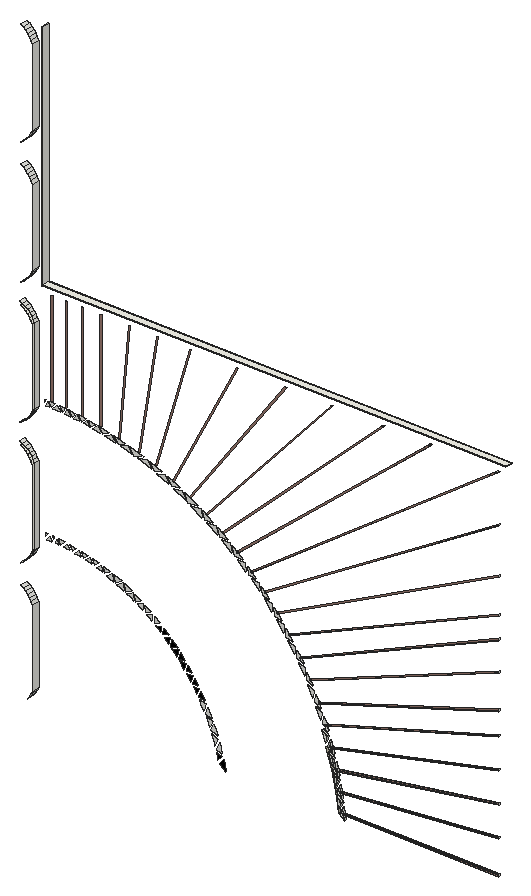
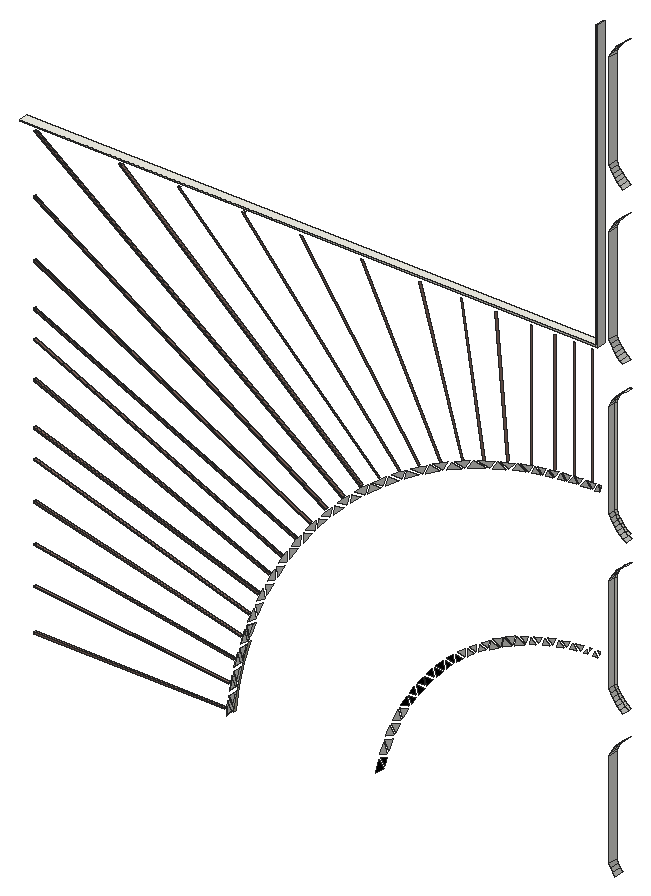
# SketchUp Ruby script. Lengths in inches.
U = 1.inch
M = Sketchup.active_model
def pt(a) = Geom::Point3d.new(a.map { |v| v * U })
def face(e, loops, mat)
  f = e.add_face(loops[0].map { |a| pt(a) })
  loops[1..].each { |l| e.add_face(l.map { |a| pt(a) }).erase! }
  f.material = f.back_material = mat if mat
  f
end
# faces: each face lists its corners as indices into pts; further lists are holes
def faces(e, pts, list, mat = nil) = list.each { |f| face(e, (f[0].is_a?(Array) ? f : [f]).map { |l| l.map { |i| pts[i] } }, mat) }
# xy, xz, yz: faces in a plane at the given z, y or x. An outline is a flat list of corners, or four numbers for a rectangle; further outlines are holes
def ring(l) = l.size == 4 ? [[l[0], l[1]], [l[2], l[1]], [l[2], l[3]], [l[0], l[3]]] : l.each_slice(2).to_a
def flat(e, list, mat, &to3) = list.each { |f| face(e, (f[0].is_a?(Array) ? f : [f]).map { |l| ring(l).map { |u, v| to3.(u, v) } }, mat) }
def xy(e, z, list, mat = nil) = flat(e, list, mat) { |x, y| [x, y, z] }
def xz(e, y, list, mat = nil) = flat(e, list, mat) { |x, z| [x, y, z] }
def yz(e, x, list, mat = nil) = flat(e, list, mat) { |y, z| [x, y, z] }
def lines(e, pts, list) = list.each { |a, b| e.add_line(pt(pts[a]), pt(pts[b])) }
# prism: a flat outline (further loops are holes) pulled along v
def prism(e, loops, v, mat = nil)
  f = face(e, loops, mat); d = Geom::Vector3d.new(v.map { |x| x * U })
  f.pushpull(f.normal.samedirection?(d) ? d.length : -d.length)
end
def box(e, o, s, mat = nil) = prism(e, [[o, [o[0] + s[0], o[1], o[2]], [o[0] + s[0], o[1] + s[1], o[2]], [o[0], o[1] + s[1], o[2]]]], [0, 0, s[2]], mat)
def at(x, y, z, deg = 0) = Geom::Transformation.translation(pt([x, y, z])) * Geom::Transformation.rotation(ORIGIN, Z_AXIS, deg.degrees)
def axes(o, x, y, z) = Geom::Transformation.new([*x, 0, *y, 0, *z, 0, *pt(o).to_a, 1])
def part(name) = M.definitions.add(name)
# library, detail: a bought-in or finely detailed component or shape, given as its bounding box
def library(name, o, s) = part(name).tap { |d| box(d.entities, o, s) }
def detail(e, o, s) = box(e.add_group.entities, o, s)
def put(e, d, t, mat = nil) = e.add_instance(d, t).tap { |i| i.material = mat if mat }
def group(e, t, mat = nil) = e.add_group.tap { |g| g.transformation = t; g.material = mat if mat }.entities
root = M.entities
M.materials.add("Tafisa-Gardenia-or-Gardenia-PM775-4K").color = [246, 245, 235]
M.materials.add("Tafisa-Terrarossa-PM780-4K").color = [148, 117, 107]
M.materials.add("Uniboard-L19-Putty-4K").color = [187, 181, 160]
M.materials.add("[Color M09]").color = [0, 0, 0]
xy(root,51.83,[[131.885,138,147.791,138.157]],"Tafisa-Terrarossa-PM780-4K")
xy(root,51.949,[[131.874,138,147.791,138.157]],"Tafisa-Terrarossa-PM780-4K")
xy(root,89.291,[[130.345,138,130.503,138.157],[135.69,138,135.862,138.157],[140.566,138,140.748,138.157],[147.588,138,147.791,138.157]])
xy(root,90,[[100.618,138,148.5,138.709]],"Uniboard-L19-Putty-4K")
xy(root,90.118,[[100.618,138,148.5,138.709]],"Tafisa-Gardenia-or-Gardenia-PM775-4K")
xz(root,138.157,[[131.8,51.347,131.745,51.932,131.653,52.513,131.327,51.879],[131.234,52.254,131.567,52.902,131.05,53.415],[119.016,52.974,118.749,53.891,118.748,53.897,118.429,53.195],[131.537,53.282,131.442,53.88,131.31,54.471,131.016,53.799],[118.288,53.48,118.6,54.168,117.933,54.514,118.219,53.719],
  [130.906,54.168,131.198,54.835,130.65,55.315],[118.539,54.477,118.344,55.018,118.178,55.401,117.877,54.82],[117.721,55.054,118.013,55.618,117.384,55.831],[131.144,55.213,131.012,55.804,130.843,56.386,130.592,55.696],[117.965,55.894,117.868,56.117,117.526,56.79,117.298,56.121],
  [130.459,56.058,130.709,56.742,130.132,57.186],[117.119,56.359,117.343,57.016,116.686,57.168,116.836,56.916],[130.631,57.115,130.462,57.697,130.257,58.267,130.049,57.563],[129.894,57.916,130.1,58.614,129.496,59.021],[130,58.982,129.795,59.552,129.554,60.108,129.391,59.392],
  [129.214,59.734,129.376,60.445,128.747,60.813],[129.252,60.805,129.012,61.361,128.737,61.901,128.619,61.176],[128.421,61.507,128.538,62.226,127.887,62.554],[128.392,62.578,128.117,63.117,127.808,63.639,127.736,62.908],[112.014,62.692,112.561,62.841,112.023,63.258],
  [111.753,62.783,111.762,63.338,111.237,63.158,111.501,62.979],[127.518,63.226,127.589,63.951,126.92,64.237],[111.069,63.378,111.605,63.562,111.043,63.944],[110.803,63.453,110.777,64.008,110.264,63.795,110.539,63.633],[109.869,63.974,109.791,64.686,109.149,64.37,109.515,64.184],
  [110.083,64.004,110.606,64.221,110.021,64.567],[127.422,64.293,127.113,64.814,126.773,65.315,126.747,64.582],[109.024,64.497,109.673,64.816,108.9,65.21],[108.848,64.524,108.725,65.229,108.104,64.874,108.481,64.71],[126.509,64.885,126.535,65.613,125.848,65.857],
  [107.971,64.992,108.6,65.351,107.803,65.696],[107.794,65.008,107.627,65.704,107.03,65.311,107.417,65.171],[106.923,65.513,107.364,65.802,106.768,66.017],[106.622,65.52,106.47,66.012,106.059,65.703,106.343,65.62],[105.51,65.862,105.328,66.344,104.937,66.009,105.226,65.945],
  [105.811,65.874,106.233,66.191,105.625,66.368],[126.346,65.944,126.005,66.445,125.634,66.923,125.654,66.19],[104.378,66.134,104.167,66.603,103.797,66.245,104.09,66.199],[104.678,66.165,105.079,66.508,104.461,66.646],[103.232,66.334,102.992,66.789,102.646,66.409,102.94,66.381],
  [103.53,66.384,103.909,66.751,103.283,66.85],[102.076,66.462,101.871,66.796,101.784,66.49],[125.397,66.477,125.377,67.205,124.677,67.406],[101.37,66.503,101.19,66.894,100.901,66.518],[102.37,66.53,102.725,66.921,102.094,66.98],
  [101.565,66.764,101.635,67.012,101.447,67.018],[100.761,66.805,100.937,67.034,100.761,67.04],[125.168,67.524,124.797,68.002,124.396,68.457,124.462,67.726],[124.188,67.997,124.123,68.722,123.411,68.878],[123.894,69.027,123.493,69.481,123.065,69.91,123.177,69.184],
  [122.886,69.4375,122.775,70.157,122.055,70.268],[122.528,70.447,122.099,70.875,121.645,71.276,121.802,70.559],[121.496,70.793,121.34,71.505,120.615,71.57],[121.157,71.743,120.638,72.2,120.06,72.648,120.321,71.819],[120.063,71.994,119.804,72.817,119.001,72.817],
  [118.79,73.011,119.593,73.011,119.079,73.409,118.555,73.766],[118.544,73.149,118.309,73.905,117.433,73.905],[117.193,74.098,118.066,74.098,117.447,74.518,117.003,74.781],[116.962,74.207,116.773,74.89,115.807,74.89],[115.513,75.083,116.493,75.083,115.749,75.523,115.133,75.837],
  [115.235,75.206,114.859,75.95,114.037,75.816],[113.78,75.97,114.607,76.105,113.991,76.419,113.356,76.693],[113.497,76.07,113.076,76.789,112.264,76.604],[111.998,76.742,112.814,76.928,112.18,77.202,111.53,77.436],[111.709,76.824,111.24,77.521,110.272,77.341],
  [109.915,77.472,110.916,77.657,110.324,77.871,109.489,78.113],[109.643,77.531,109.228,78.157,108.553,77.848],[108.305,77.947,108.986,78.259,108.429,78.421,107.814,78.558],[108.029,77.982,107.541,78.59,106.886,78.238],[106.651,78.331,107.292,78.675,106.503,78.851,106.359,78.874],
  [106.427,78.34,106.151,78.852,105.664,78.462,106.407,78.345],[105.271,78.525,105.052,79.006,104.677,78.619],[105.47,78.554,105.951,78.939,105.244,79.051],[104.29,78.667,103.991,79.138,103.692,78.724],[104.494,78.708,104.883,79.108,104.555,79.16,104.184,79.195],
  [103.308,78.76,102.956,79.234,102.712,78.817],[103.514,78.807,103.819,79.23,103.154,79.292],[102.344,78.838,101.957,79.315,101.541,78.863],[101.168,78.875,100.971,79.269,100.774,78.887],[102.539,78.904,102.787,79.327,102.59,79.346,102.17,79.359],
  [101.351,78.942,101.747,79.372,101.325,79.385,101.129,79.385],[100.715,79.193,100.814,79.385,100.715,79.385]])
xz(root,138.157,[[131.885,51.83,147.791,51.83,147.791,51.949,131.874,51.949],[131.583,53.786,147.791,55.307,147.791,55.426,131.564,53.903],[131.159,55.719,147.791,58.431,147.791,58.551,131.133,55.835],[130.614,57.622,147.791,61.594,147.791,61.716,130.581,57.735],[129.95,59.486,147.791,64.758,147.791,64.881,129.91,59.598],
  [129.171,61.305,147.791,67.121,147.791,67.244,129.124,61.414],[128.279,63.072,147.791,70.662,147.791,70.788,128.226,63.177],[127.279,64.778,147.791,73.694,147.791,73.823,127.218,64.881],[126.106,66.518,147.791,75.943,147.791,76.072,147.744,76.051,126.059,66.626,126.031,66.614],[124.893,68.082,147.791,79.556,147.791,79.689,147.738,79.662,124.84,68.187,124.812,68.173],
  [123.584,69.566,147.791,84.298,147.791,84.436,147.73,84.398,123.522,69.667,123.498,69.652],[122.184,70.966,147.791,89.291,147.588,89.291,122.116,71.062,122.093,71.046],[120.7,72.275,140.748,89.291,140.566,89.291,120.623,72.365,120.604,72.349],[119.136,73.488,135.862,89.291,135.69,89.291,119.055,73.573,119.036,73.556],[117.499,74.6,130.503,89.291,130.345,89.291,117.411,74.678,117.395,74.661],
  [115.795,75.607,125.683,89.291,125.537,89.291,115.7,75.677,115.689,75.662],[114.032,76.506,120.629,89.291,120.497,89.291,113.936,76.575,113.925,76.552],[112.216,77.292,115.795,89.291,115.674,89.291,112.111,77.346,112.106,77.331],[110.467,77.922,110.47,77.943,112.332,89.272,112.335,89.291,112.216,89.291,110.353,77.962],[108.453,78.515,109.469,89.291,109.35,89.291,108.337,78.541],
  [106.521,78.946,106.521,89.291,106.403,89.291,106.403,78.965],[104.567,79.256,104.567,89.291,104.449,89.291,104.449,79.267],[102.947,79.409,102.947,89.291,102.829,89.291,102.829,79.42],[101.445,79.478,101.445,89.291,101.327,89.291,101.327,79.482]],"Tafisa-Terrarossa-PM780-4K")
xz(root,138.157,[[119.36,51.478,119.345,51.572,119.136,52.505,118.724,52.022],[118.617,52.275,118.995,52.719,118.45,52.924,118.543,52.602],[117.264,57.287,116.838,58.007,116.603,57.44],[116.415,57.628,116.638,58.166,116.055,58.194,116.244,57.916],[116.533,58.441,116.187,58.95,116.018,58.465],
  [115.788,58.534,116.01,59.169,115.327,59.169,115.566,58.861],[115.333,59.408,115.855,59.408,115.478,59.894],[115.099,59.463,115.277,60.058,114.608,60.058,114.855,59.778],[114.581,60.298,115.148,60.298,114.689,60.819],[114.348,60.353,114.487,61.024,113.809,60.927,114.087,60.648],
  [113.721,61.103,114.407,61.201,113.819,61.789],[113.518,61.271,113.596,61.821,113.053,61.708,113.293,61.497],[112.914,61.947,113.469,62.062,112.959,62.512],[112.659,62.055,112.703,62.608,112.168,62.462,112.42,62.266]],"[Color M09]")
xz(root,138.709,[[100.5,90,100.618,114],[100.618,90,148.5,90.118]],"Tafisa-Gardenia-or-Gardenia-PM775-4K")
yz(root,99.5,[[138,52,138.787,60],[138.25,65,138.787,73],[138.25,78,138.787,86],[138,91,138.787,99],[138,104,138.787,112]])
yz(root,99.5,[[138,65,138.25,73],[138,78,138.25,86]],"Tafisa-Gardenia-or-Gardenia-PM775-4K")
yz(root,100.5,[[138,90,138.709,114]])
yz(root,100.618,[[138,90.118,138.709,114]])
yz(root,147.791,[[138,51.83,138.157,51.949],[138,55.307,138.157,55.426],[138,58.431,138.157,58.551],[138,61.594,138.157,61.716],[138,64.758,138.157,64.881],
  [138,67.121,138.157,67.244],[138,70.662,138.157,70.788],[138,73.694,138.157,73.823],[138,75.943,138.157,76.072],[138,79.556,138.157,79.689],
  [138,84.298,138.157,84.436]])
p = [[99.206,138.787,51.441],[99.019,138.787,51.185],[99.019,138,51.185],[99.206,138,51.441],[131.327,138,51.879],[131.8,138,51.347],
  [131.8,138.157,51.347],[131.327,138.157,51.879],[131.745,138,51.932],[131.745,138.157,51.932],[99.367,138.787,51.713],[99.367,138,51.713],
  [99.5,138.787,52],[99.5,138,52],[131.874,138,51.949],[131.885,138,51.83],[131.885,138.157,51.83],[131.874,138.157,51.949],
  [131.171,138,51.86],[130.868,138,53.77],[130.868,138.157,53.77],[131.171,138.157,51.86],[131.653,138,52.513],[131.653,138.157,52.513],
  [131.05,138,53.415],[131.234,138,52.254],[131.234,138.157,52.254],[131.05,138.157,53.415],[131.567,138,52.902],[131.567,138.157,52.902],
  [131.016,138,53.799],[131.537,138,53.282],[131.537,138.157,53.282],[131.016,138.157,53.799],[131.442,138,53.88],[131.442,138.157,53.88],
  [130.446,138,55.658],[130.446,138.157,55.658],[131.31,138,54.471],[131.31,138.157,54.471],[131.564,138,53.903],[131.583,138,53.786],
  [131.583,138.157,53.786],[131.564,138.157,53.903],[147.791,138,55.307],[147.791,138.157,55.307],[147.791,138,55.426],[147.791,138.157,55.426],
  [130.65,138,55.315],[130.906,138,54.168],[130.906,138.157,54.168],[130.65,138.157,55.315],[131.198,138,54.835],[131.198,138.157,54.835],
  [130.592,138,55.696],[131.144,138,55.213],[131.144,138.157,55.213],[130.592,138.157,55.696],[131.012,138,55.804],[131.012,138.157,55.804],
  [129.906,138,57.516],[129.906,138.157,57.516],[130.843,138,56.386],[130.843,138.157,56.386],[131.133,138,55.835],[131.159,138,55.719],
  [131.159,138.157,55.719],[131.133,138.157,55.835],[147.791,138,58.431],[147.791,138.157,58.431],[147.791,138,58.551],[147.791,138.157,58.551],
  [130.132,138,57.186],[130.459,138,56.058],[130.459,138.157,56.058],[130.132,138.157,57.186],[130.709,138,56.742],[130.709,138.157,56.742],
  [130.049,138,57.563],[130.631,138,57.115],[130.631,138.157,57.115],[130.049,138.157,57.563],[130.462,138,57.697],[130.462,138.157,57.697],
  [130.257,138,58.267],[130.257,138.157,58.267],[130.581,138,57.735],[130.614,138,57.622],[130.614,138.157,57.622],[130.581,138.157,57.735],
  [147.791,138,61.594],[147.791,138.157,61.594],[147.791,138,61.716],[147.791,138.157,61.716],[129.496,138,59.021],[129.894,138,57.916],
  [129.894,138.157,57.916],[129.496,138.157,59.021],[130.1,138,58.614],[130.1,138.157,58.614],[130,138,58.982],[129.795,138,59.552],
  [129.795,138.157,59.552],[130,138.157,58.982],[129.91,138,59.598],[129.95,138,59.486],[129.95,138.157,59.486],[129.91,138.157,59.598],
  [147.791,138,64.758],[147.791,138.157,64.758],[147.791,138,64.881],[147.791,138.157,64.881],[99.367,138.787,60.287],[99.5,138.787,60],
  [99.5,138,60],[99.367,138,60.287],[99.206,138.787,60.559],[99.206,138,60.559],[99.019,138.787,60.815],[99.019,138,60.815],
  [98.808,138.787,61.05],[98.808,138,61.05],[98.574,138.787,61.264],[98.574,138,61.264],[98.321,138.787,61.453],[98.321,138,61.453],
  [129.171,138,61.305],[147.791,138,67.121],[147.791,138.157,67.121],[129.171,138.157,61.305],[147.791,138,67.244],[129.124,138,61.414],
  [129.124,138.157,61.414],[147.791,138.157,67.244],[128.279,138,63.072],[147.791,138,70.662],[147.791,138.157,70.662],[128.279,138.157,63.072],
  [147.791,138,70.788],[128.226,138,63.177],[128.226,138.157,63.177],[147.791,138.157,70.788],[98.321,138,63.547],[98.574,138,63.736],
  [98.574,138.25,63.736],[98.321,138.25,63.547],[98.574,138.787,63.736],[98.321,138.787,63.547],[98.808,138,63.95],[98.808,138.25,63.95],
  [98.808,138.787,63.95],[99.019,138,64.185],[99.019,138.25,64.185],[99.019,138.787,64.185],[99.206,138,64.441],[99.206,138.25,64.441],
  [99.206,138.787,64.441],[99.367,138,64.713],[99.367,138.25,64.713],[99.367,138.787,64.713],[99.5,138,65],[99.5,138.25,65],
  [99.5,138.787,65],[127.279,138,64.778],[147.791,138,73.694],[147.791,138.157,73.694],[127.279,138.157,64.778],[147.791,138,73.823],
  [127.218,138,64.881],[127.218,138.157,64.881],[147.791,138.157,73.823],[126.106,138,66.518],[147.791,138,75.943],[147.791,138.157,75.943],
  [126.106,138.157,66.518],[147.744,138,76.051],[126.059,138,66.626],[126.059,138.157,66.626],[147.744,138.157,76.051],[124.893,138,68.082],
  [147.791,138,79.556],[147.791,138.157,79.556],[124.893,138.157,68.082],[147.738,138,79.662],[124.84,138,68.187],[124.84,138.157,68.187],
  [147.738,138.157,79.662],[123.584,138,69.566],[147.791,138,84.298],[147.791,138.157,84.298],[123.584,138.157,69.566],[147.73,138,84.398],
  [123.522,138,69.667],[123.522,138.157,69.667],[147.73,138.157,84.398],[122.184,138,70.966],[147.791,138,89.291],[147.791,138.157,89.291],
  [122.184,138.157,70.966],[147.588,138,89.291],[122.116,138,71.062],[122.116,138.157,71.062],[147.588,138.157,89.291],[120.7,138,72.275],
  [140.748,138,89.291],[140.748,138.157,89.291],[120.7,138.157,72.275],[140.566,138,89.291],[120.623,138,72.365],[120.623,138.157,72.365],
  [140.566,138.157,89.291],[99.5,138,73],[99.367,138,73.287],[99.367,138.25,73.287],[99.5,138.25,73],[99.367,138.787,73.287],
  [99.5,138.787,73],[99.206,138,73.559],[99.206,138.25,73.559],[99.206,138.787,73.559],[99.019,138,73.815],[99.019,138.25,73.815],
  [99.019,138.787,73.815],[98.808,138,74.05],[98.808,138.25,74.05],[98.808,138.787,74.05],[98.574,138,74.264],[98.574,138.25,74.264],
  [98.574,138.787,74.264],[98.321,138,74.453],[98.321,138.25,74.453],[98.321,138.787,74.453],[98.05,138.787,74.617],[98.05,138.25,74.617],
  [147.791,138,76.072],[147.791,138.157,76.072],[98.321,138.787,76.547],[98.05,138.787,76.383],[98.05,138.25,76.383],[98.321,138.25,76.547],
  [98.321,138,76.547],[98.574,138,76.736],[98.574,138.25,76.736],[98.574,138.787,76.736],[98.808,138,76.95],[98.808,138.25,76.95],
  [98.808,138.787,76.95],[99.019,138,77.185],[99.019,138.25,77.185],[99.019,138.787,77.185],[99.206,138,77.441],[99.206,138.25,77.441],
  [99.206,138.787,77.441],[99.367,138,77.713],[99.367,138.25,77.713],[99.367,138.787,77.713],[99.5,138,78],[99.5,138.25,78],
  [99.5,138.787,78],[147.791,138,79.689],[147.791,138.157,79.689],[147.791,138,84.436],[147.791,138.157,84.436],[99.5,138,86],
  [99.367,138,86.287],[99.367,138.25,86.287],[99.5,138.25,86],[99.367,138.787,86.287],[99.5,138.787,86],[99.206,138,86.559],
  [99.206,138.25,86.559],[99.206,138.787,86.559],[99.019,138,86.815],[99.019,138.25,86.815],[99.019,138.787,86.815],[98.808,138,87.05],
  [98.808,138.25,87.05],[98.808,138.787,87.05],[98.574,138,87.264],[98.574,138.25,87.264],[98.574,138.787,87.264],[98.321,138,87.453],
  [98.321,138.25,87.453],[98.321,138.787,87.453],[98.05,138.787,87.617],[98.05,138.25,87.617],[98.574,138.787,89.736],[98.321,138.787,89.547],
  [98.321,138,89.547],[98.574,138,89.736],[98.808,138.787,89.95],[98.808,138,89.95],[99.019,138.787,90.185],[99.019,138,90.185],
  [99.206,138.787,90.441],[99.206,138,90.441],[99.367,138.787,90.713],[99.367,138,90.713],[99.5,138.787,91],[99.5,138,91],
  [99.367,138.787,99.287],[99.5,138.787,99],[99.5,138,99],[99.367,138,99.287],[99.206,138.787,99.559],[99.206,138,99.559],
  [99.019,138.787,99.815],[99.019,138,99.815],[98.808,138.787,100.05],[98.808,138,100.05],[98.574,138.787,100.264],[98.574,138,100.264],
  [98.321,138.787,100.453],[98.321,138,100.453],[98.574,138.787,102.736],[98.321,138.787,102.547],[98.321,138,102.547],[98.574,138,102.736],
  [98.808,138.787,102.95],[98.808,138,102.95],[99.019,138.787,103.185],[99.019,138,103.185],[99.206,138.787,103.441],[99.206,138,103.441],
  [99.367,138.787,103.713],[99.367,138,103.713],[99.5,138.787,104],[99.5,138,104],[99.367,138.787,112.287],[99.5,138.787,112],
  [99.5,138,112],[99.367,138,112.287],[99.206,138.787,112.559],[99.206,138,112.559],[99.019,138.787,112.815],[99.019,138,112.815],
  [98.808,138.787,113.05],[98.808,138,113.05],[98.574,138.787,113.264],[98.574,138,113.264],[98.321,138.787,113.453],[98.321,138,113.453]]
faces(root,p,[[0,1,2,3],[4,5,6,7],[5,8,9,6],[10,0,3,11],[12,10,11,13],[14,15,16,17],[22,4,7,23],[8,22,23,9],
  [24,25,26,27],[25,28,29,26],[28,24,27,29],[30,31,32,33],[31,34,35,32],[38,30,33,39],[40,41,42,43],[34,38,39,35],
  [48,49,50,51],[49,52,53,50],[52,48,51,53],[54,55,56,57],[55,58,59,56],[62,54,57,63],[64,65,66,67],[58,62,63,59],
  [72,73,74,75],[73,76,77,74],[76,72,75,77],[78,79,80,81],[79,82,83,80],[84,78,81,85],[86,87,88,89],[82,84,85,83],
  [94,95,96,97],[95,98,99,96],[98,94,97,99],[100,101,102,103],[104,105,106,107],[112,113,114,115],[116,112,115,117],[118,116,117,119],
  [120,118,119,121],[122,120,121,123],[124,122,123,125],[146,147,145,144],[150,146,144,149],[153,150,149,152],[156,153,152,155],[159,156,155,158],
  [162,159,158,161],[215,216,214,213],[219,215,213,218],[222,219,218,221],[225,222,221,224],[228,225,224,227],[231,228,227,230],[232,231,230,233],
  [234,175,178,235],[236,237,238,239],[243,236,239,242],[246,243,242,245],[249,246,245,248],[252,249,248,251],[255,252,251,254],[258,255,254,257],
  [259,183,186,260],[267,268,266,265],[271,267,265,270],[274,271,270,273],[277,274,273,276],[280,277,276,279],[283,280,279,282],[284,283,282,285],
  [286,287,288,289],[290,286,289,291],[292,290,291,293],[294,292,293,295],[296,294,295,297],[298,296,297,299],[300,301,302,303],[304,300,303,305],
  [306,304,305,307],[308,306,307,309],[310,308,309,311],[312,310,311,313],[314,315,316,317],[318,314,317,319],[320,318,319,321],[322,320,321,323],
  [324,322,323,325],[326,324,325,327],[328,329,330,331],[332,328,331,333],[334,332,333,335],[336,334,335,337],[338,336,337,339],[340,338,339,341]])
faces(root,p,[[18,19,20,21],[19,36,37,20],[36,60,61,37]],"Uniboard-L19-Putty-4K")
faces(root,p,[[41,44,45,42],[46,40,43,47],[65,68,69,66],[70,64,67,71],[87,90,91,88],[92,86,89,93],[105,108,109,106],[110,104,107,111],
  [126,127,128,129],[130,131,132,133],[134,135,136,137],[138,139,140,141],[163,164,165,166],[167,168,169,170],[171,172,173,174],[175,176,177,178],
  [179,180,181,182],[183,184,185,186],[187,188,189,190],[191,192,193,194],[195,196,197,198],[199,200,201,202],[203,204,205,206],[207,208,209,210],
  [261,191,194,262]],"Tafisa-Terrarossa-PM780-4K")
faces(root,p,[[142,143,144,145],[143,148,149,144],[148,151,152,149],[151,154,155,152],[154,157,158,155],[157,160,161,158],[211,212,213,214],[212,217,218,213],
  [217,220,221,218],[220,223,224,221],[223,226,227,224],[226,229,230,227],[240,241,242,239],[241,244,245,242],[244,247,248,245],[247,250,251,248],
  [250,253,254,251],[253,256,257,254],[263,264,265,266],[264,269,270,265],[269,272,273,270],[272,275,276,273],[275,278,279,276],[278,281,282,279]],"Tafisa-Gardenia-or-Gardenia-PM775-4K")
